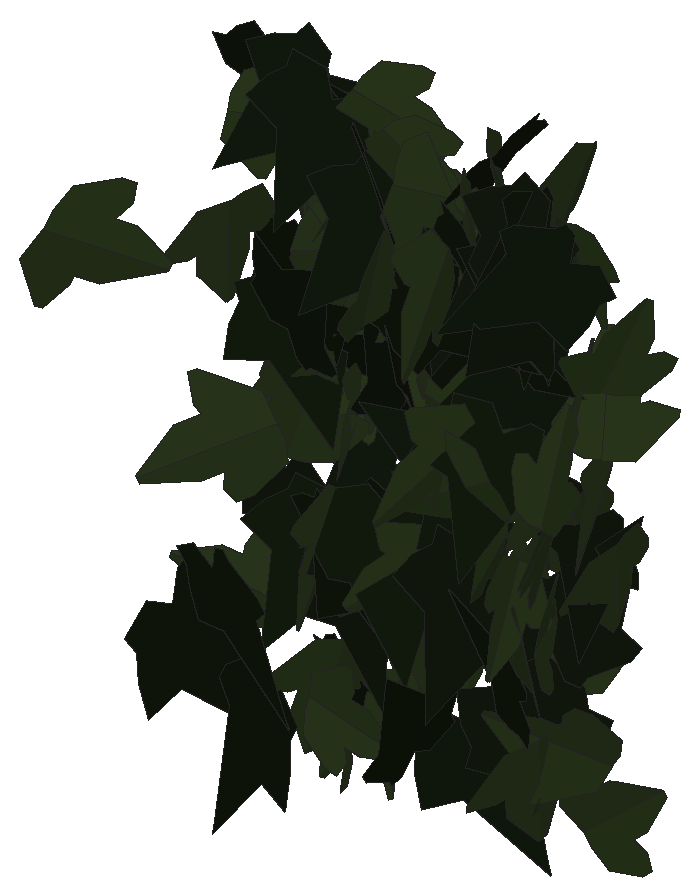
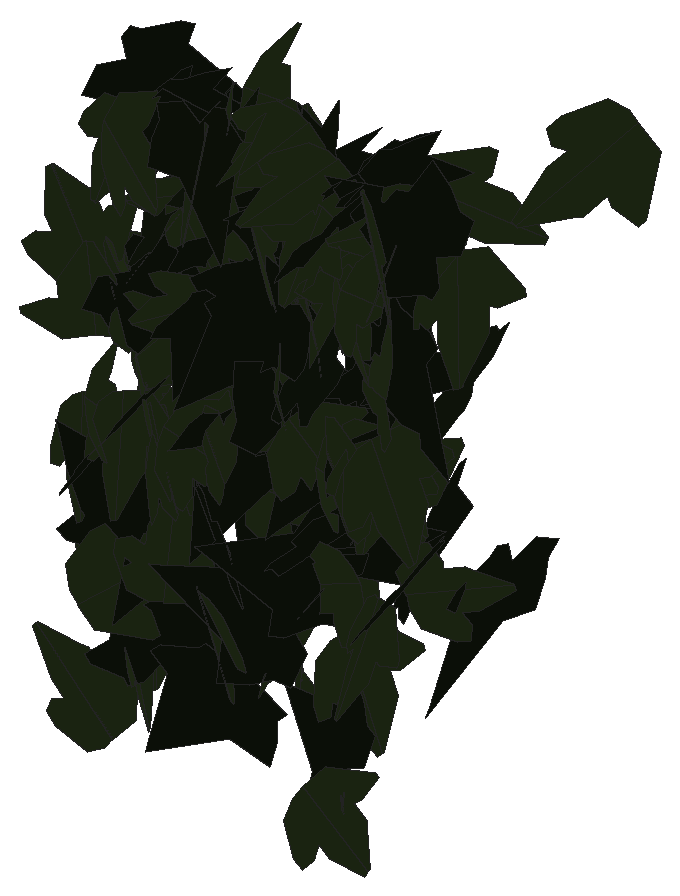
# SketchUp Ruby script. Lengths in inches.
U = 1.inch
M = Sketchup.active_model
def pt(a) = Geom::Point3d.new(a.map { |v| v * U })
def face(e, loops, mat)
  f = e.add_face(loops[0].map { |a| pt(a) })
  loops[1..].each { |l| e.add_face(l.map { |a| pt(a) }).erase! }
  f.material = f.back_material = mat if mat
  f
end
# faces: each face lists its corners as indices into pts; further lists are holes
def faces(e, pts, list, mat = nil) = list.each { |f| face(e, (f[0].is_a?(Array) ? f : [f]).map { |l| l.map { |i| pts[i] } }, mat) }
# xy, xz, yz: faces in a plane at the given z, y or x. An outline is a flat list of corners, or four numbers for a rectangle; further outlines are holes
def ring(l) = l.size == 4 ? [[l[0], l[1]], [l[2], l[1]], [l[2], l[3]], [l[0], l[3]]] : l.each_slice(2).to_a
def flat(e, list, mat, &to3) = list.each { |f| face(e, (f[0].is_a?(Array) ? f : [f]).map { |l| ring(l).map { |u, v| to3.(u, v) } }, mat) }
def xy(e, z, list, mat = nil) = flat(e, list, mat) { |x, y| [x, y, z] }
def xz(e, y, list, mat = nil) = flat(e, list, mat) { |x, z| [x, y, z] }
def yz(e, x, list, mat = nil) = flat(e, list, mat) { |y, z| [x, y, z] }
def lines(e, pts, list) = list.each { |a, b| e.add_line(pt(pts[a]), pt(pts[b])) }
# prism: a flat outline (further loops are holes) pulled along v
def prism(e, loops, v, mat = nil)
  f = face(e, loops, mat); d = Geom::Vector3d.new(v.map { |x| x * U })
  f.pushpull(f.normal.samedirection?(d) ? d.length : -d.length)
end
def box(e, o, s, mat = nil) = prism(e, [[o, [o[0] + s[0], o[1], o[2]], [o[0] + s[0], o[1] + s[1], o[2]], [o[0], o[1] + s[1], o[2]]]], [0, 0, s[2]], mat)
def at(x, y, z, deg = 0) = Geom::Transformation.translation(pt([x, y, z])) * Geom::Transformation.rotation(ORIGIN, Z_AXIS, deg.degrees)
def axes(o, x, y, z) = Geom::Transformation.new([*x, 0, *y, 0, *z, 0, *pt(o).to_a, 1])
def part(name) = M.definitions.add(name)
# library, detail: a bought-in or finely detailed component or shape, given as its bounding box
def library(name, o, s) = part(name).tap { |d| box(d.entities, o, s) }
def detail(e, o, s) = box(e.add_group.entities, o, s)
def put(e, d, t, mat = nil) = e.add_instance(d, t).tap { |i| i.material = mat if mat }
def group(e, t, mat = nil) = e.add_group.tap { |g| g.transformation = t; g.material = mat if mat }.entities
root = M.entities
M.materials.add("efeu1").color = [18, 25, 13]
M.materials.add("efeu2").color = [43, 57, 29]
c1 = part("ivyleaf_10")
p = [[0,0.5,-0.03],[-0.0625,2.02,-0.43],[-0.19,2.01,-0.46],[-0.54,1.05,-0.29],[-0.52,0.625,-0.18],[-0.83,0.76,-0.28],
  [-1.16,0.64,-0.33],[-1.15,0.33,-0.24],[-0.77,-0.39,0.02],[-0.3,-0.51,0.16],[0.04,-0.48,0.23],[-0.02,2.01,-0.4375],
  [-0.06,2.01,-0.43],[0.04,-0.49,0.23],[0.67,-0.49,0.14],[1.38,0.36,-0.2],[1.375,0.51,-0.24],[0.81,0.65,-0.19],
  [0.62,0.59,-0.15],[0.6,1.09,-0.28],[0.5,1.23,-0.31]]
faces(c1.entities,p,[[0,1,2,3,4,5,6,7,8,9,10],[11,12,0,13,14,15,16,17,18,19,20]],"efeu2")
c2 = part("ivyleaf_9")
p = [[1.54,2.16,1.25],[1.36,2.04,1.19],[-0.21,0.99,0.68],[-0.71,1.11,0.82],[-0.85,0.86,0.67],[-0.8,0.17,0.21],
  [-0.9,-0.01,0.1],[-0.67,-0.16,-0.02],[-0.08,-0.08,-0.05],[-0.03,-0.6,-0.4],[0.65,-0.88,-0.66],[0.83,-0.6,-0.49],
  [1.29,-0.42,-0.43],[1.8125,-0.07,-0.26],[1.21,0.44,0.15]]
faces(c2.entities,p,[[0,1,2,3,4,5,6,7,8,9,10,11,12,13,14]],"efeu1")
put(root,c1,axes([527.41,129.42,180.43],[-0.32518,-0.15247,0.84845],[-0.53013,-0.67969,-0.32533],[0.67976,-0.60302,0.15216]))
put(root,c2,axes([526.49,129.75,177.46],[0.55857,-0.71655,0.03403],[0.02142,-0.02645,-0.90854],[0.71704,0.55898,0.00063]))
put(root,c2,axes([526.71,130.62,174.9],[0.21927,-0.17934,-0.93924],[0.70617,-0.61934,0.28311],[-0.64472,-0.73937,-0.00933]))
put(root,c1,axes([523.77,129.47,182.67],[-0.35518,-0.42275,-0.82011],[0.53108,0.62493,-0.55215],[0.75449,-0.6389,0.00258]))
put(root,c1,axes([529.14,131.85,182.77],[-0.01286,-0.49305,0.76391],[0.44109,-0.67144,-0.42595],[0.79505,0.36454,0.24867]))
put(root,c2,axes([528.87,131.65,174.39],[0.24289,0.34244,0.63851],[-0.35118,-0.5334,0.41966],[0.63374,-0.42682,-0.01217]))
put(root,c1,axes([529.3,132.11,179.68],[-0.03772,-0.35118,0.79561],[0.03726,-0.79628,-0.34971],[0.86887,0.0189,0.04954]))
put(root,c2,axes([524.5,131.26,175.47],[0.28969,-0.5067,-0.76251],[-0.37111,0.66613,-0.58364],[0.83693,0.47076,0.00513]))
put(root,c1,axes([529.81,131.96,179.26],[-0.41254,-0.12179,0.76212],[-0.73922,-0.18605,-0.42987],[0.22185,-0.84641,-0.01517]))
put(root,c1,axes([526.91,131.92,174.23],[0.1049,0.03854,0.74126],[0.72695,0.14594,-0.11046],[-0.14999,0.73428,-0.01695]))
put(root,c1,axes([527.66,132.14,181.54],[0.01458,-0.75101,-0.08197],[0.00317,-0.08192,0.75115],[-0.75546,-0.01484,0.00157]))
put(root,c2,axes([529.8,132.64,179.75],[-0.34229,-0.72229,-0.01541],[0.00393,0.01519,-0.79928],[0.72244,-0.3423,-0.00295]))
put(root,c1,axes([530.18,132.5625,177.34],[0.0409,0.59628,-0.475],[-0.03328,-0.47383,-0.59769],[-0.76162,0.05273,0.00061]))
put(root,c1,axes([526.38,132.72,177.13],[0.20032,-0.68078,0.51492],[0.26377,-0.45365,-0.70239],[0.81181,0.31539,0.10116]))
put(root,c2,axes([530.94,132.8125,183.15],[-0.03571,-0.07267,-0.76744],[-0.13202,-0.75633,0.07776],[-0.75948,0.13489,0.02257]))
put(root,c2,axes([529.05,132.98,176.75],[-0.1738,-0.80386,0.29707],[-0.05274,-0.29251,-0.82238],[0.85538,-0.18137,0.00965]))
put(root,c1,axes([525.05,132.65,175.39],[0.19656,0.13798,0.69312],[-0.57621,-0.38526,0.2401],[0.40919,-0.60879,0.00515]))
put(root,c2,axes([529.85,133.16,181.98],[-0.20965,-0.53927,0.62119],[0.02087,-0.64433,-0.55231],[0.82235,-0.12113,0.17239]))
put(root,c2,axes([530.07,132.68,175.26],[0.21332,-0.68005,0.27052],[-0.05728,0.2654,0.71235],[-0.72964,-0.21966,0.02316]))
put(root,c2,axes([526.27,133.19,176.25],[-0.07891,-0.48877,0.70375],[0.14001,-0.70458,-0.47365],[0.84531,0.07108,0.14414]))
put(root,c2,axes([527.08,133.25,182.48],[-0.34583,-0.60775,0.4634],[-0.12688,-0.45592,-0.69263],[0.75365,-0.35563,0.09603]))
put(root,c2,axes([525.41,132.92,180.11],[-0.25145,0.02371,0.8195],[0.4664,-0.70082,0.16338],[0.67426,0.49362,0.1926]))
put(root,c1,axes([530.21,132.75,175.6],[-0.67654,0.37459,0.1769],[0.15072,-0.09297,0.77328],[0.38587,0.69308,0.00812]))
put(root,c1,axes([527.69,133.32,176.61],[-0.05182,-0.31934,0.67271],[-0.16909,-0.65167,-0.32238],[0.7252,-0.17477,-0.02709]))
put(root,c2,axes([527.92,132.6,181.71],[0.1428,0.07843,-0.84206],[0.61962,0.57151,0.1583],[0.57558,-0.63469,0.03849]))
put(root,c1,axes([530.5625,132.86,178.17],[0.30633,-0.69715,-0.10742],[-0.04415,0.09793,-0.76148],[0.70399,0.30949,-0.00102]))
put(root,c1,axes([530.85,132.39,179.09],[0.03357,0.59128,-0.48542],[0.04784,0.48331,0.59202],[0.76351,-0.05628,-0.01575]))
put(root,c2,axes([527.09,133.43,180.13],[0.06108,-0.26606,0.77227],[0.17975,-0.75106,-0.27297],[0.79679,0.18983,0.00239]))
put(root,c1,axes([529.98,133.47,178.53],[-0.04596,0.19222,0.7632],[0.13301,-0.75161,0.19731],[0.77572,0.14026,0.01138]))
put(root,c2,axes([528.67,133.44,182.21],[0.15351,-0.58562,0.55405],[0.21399,-0.51418,-0.60276],[0.77726,0.25722,0.05652]))
put(root,c1,axes([524.18,132.92,181.58],[-0.25348,-0.82349,-0.10141],[0.03287,0.09598,-0.86161],[0.82906,-0.25558,0.00316]))
put(root,c2,axes([527.25,133.14,177.23],[-0.3073,-0.7536,-0.39936],[0.16105,0.36559,-0.81379],[0.83754,-0.34681,0.00995]))
put(root,c2,axes([529.86,133.56,183.02],[-0.42279,-0.51969,0.3609],[-0.1893,-0.31028,-0.66856],[0.60374,-0.46123,0.04311]))
put(root,c1,axes([530.76,132.52,176.46],[-0.02787,0.11799,0.75725],[-0.52626,0.54791,-0.10474],[-0.55714,-0.52345,0.06105]))
put(root,c1,axes([530.24,132.96,174.125],[-0.23443,-0.86981,-0.17617],[0.02648,0.17527,-0.90063],[0.88708,-0.2351,-0.01967]))
put(root,c2,axes([525.73,133.53,176.4],[-0.45283,-0.61602,0.09287],[-0.04067,-0.08533,-0.76435],[0.62165,-0.45432,0.01764]))
put(root,c1,axes([530.87,133.42,174.13],[-0.4028,-0.0512,-0.76261],[-0.69714,-0.32881,0.39029],[-0.31337,0.79731,0.11198]))
put(root,c2,axes([526.57,133.63,182.68],[0.13874,-0.35581,0.72277],[0.23203,-0.68469,-0.3816],[0.77147,0.26991,-0.01521]))
put(root,c1,axes([526,133.34,174.21],[-0.25301,-0.79026,0.19399],[-0.03494,-0.19241,-0.8294],[0.81297,-0.25421,0.02473]))
put(root,c2,axes([526.18,133.42,175.75],[0.26533,-0.75038,-0.0322],[-0.00195,0.03346,-0.79585],[0.75107,0.26517,0.00931]))
put(root,c1,axes([526.82,133.52,173.66],[0.51984,-0.21967,0.46904],[0.42379,-0.20163,-0.56412],[0.29775,0.6705,-0.01597]))
put(root,c2,axes([529.6875,133.93,182.85],[0.07526,-0.24162,-0.73314],[0.37389,-0.63303,0.24701],[-0.67534,-0.3774,0.05505]))
put(root,c1,axes([528.3,133.7,182.87],[0.17681,-0.2807,0.67421],[0.59399,-0.3483,-0.30079],[0.42489,0.60374,0.13994]))
put(root,c2,axes([525.36,133.95,183.55],[-0.25212,-0.72096,0.24078],[-0.04237,-0.23995,-0.76286],[0.75892,-0.25291,0.0374]))
put(root,c1,axes([530.09,133.48,178.02],[0.39837,-0.81768,-0.10342],[-0.03728,0.09687,-0.90952],[0.82335,0.40002,0.00886]))
put(root,c1,axes([525.07,133.48,177.73],[-0.60973,-0.62896,0.18263],[0.12417,0.13398,0.87599],[-0.64306,0.62224,-0.00402]))
put(root,c1,axes([528.7,134.01,177],[-0.03987,-0.04323,0.82819],[0.48947,-0.67056,-0.01144],[0.66947,0.48769,0.05769]))
put(root,c1,axes([526.31,133.45,180.84],[-0.6053,-0.5947,0.31322],[0.22714,0.21573,0.84855],[-0.6326,0.6465,0.00498]))
put(root,c2,axes([524.96,134.18,183.64],[-0.35741,-0.50814,0.46153],[-0.27861,-0.36817,-0.62111],[0.62737,-0.45299,-0.0129]))
put(root,c2,axes([528.25,133.31,180.88],[0.07932,0.10384,-0.80539],[0.4976,0.63329,0.13066],[0.64174,-0.50388,-0.00176]))
put(root,c2,axes([524.9,133.77,180.03],[-0.1353,-0.70648,-0.3928],[0.14631,0.37029,-0.71638],[0.79498,-0.18839,0.06499]))
put(root,c1,axes([527.58,133.17,183.21],[0.06778,-0.45707,-0.70584],[0.35803,0.65642,-0.39069],[0.76088,-0.26816,0.24671]))
put(root,c2,axes([529.72,134.21,180.31],[-0.06714,-0.08179,-0.85804],[-0.24143,-0.8244,0.09748],[-0.82743,0.24718,0.04119]))
put(root,c1,axes([527.02,133.7,183.54],[-0.54247,-0.07339,-0.4915],[0.49257,0.01699,-0.54618],[0.06584,-0.73181,0.03661]))
put(root,c1,axes([527.64,133.72,179.75],[0.66039,-0.34254,0.078],[-0.05548,0.0623,0.74336],[-0.3469,-0.66206,0.0296]))
put(root,c2,axes([528.98,134.31,181.7],[0.22256,-0.64511,0.45029],[0.17516,-0.41559,-0.68196],[0.76697,0.28211,0.02508]))
put(root,c2,axes([528.39,134.26,177.61],[-0.26693,-0.84508,-0.18534],[-0.05178,-0.17801,0.88623],[-0.86361,0.27188,0.00415]))
put(root,c2,axes([525.07,133.77,180.64],[0.24414,0.10742,-0.85145],[-0.78577,-0.32795,-0.26668],[-0.34506,0.82281,0.00487]))
put(root,c1,axes([528.6,133.8,182],[-0.25106,-0.13216,-0.68773],[0.69984,-0.02029,-0.25158],[0.02593,-0.73184,0.13117]))
put(root,c1,axes([530.26,133.73,179.28],[0.47243,-0.64562,0.27146],[-0.16721,0.21399,0.79996],[-0.68011,-0.50108,-0.00812]))
put(root,c1,axes([527.11,133.85,173.92],[-0.20857,0.73523,0.02383],[-0.02107,-0.03073,0.76371],[0.73531,0.20767,0.02865]))
put(root,c2,axes([524.32,134.21,176.51],[0.27125,-0.75607,0.00052],[0.00011,-0.00051,-0.80326],[0.75607,0.27125,-0.00007]))
put(root,c2,axes([527.81,133.59,177.88],[0.65273,0.46953,-0.12028],[-0.10145,-0.06494,-0.80403],[-0.47396,0.66053,0.00645]))
put(root,c1,axes([529.9375,134.02,173.55],[0.28991,-0.71346,-0.09655],[-0.03309,0.09078,-0.77011],[0.7192,0.29178,0.00349]))
put(root,c1,axes([525.49,134.22,178.6],[0.48937,0.15099,-0.52077],[-0.49645,-0.15732,-0.51212],[-0.21803,0.69709,-0.00278]))
put(root,c1,axes([527.15,134.22,181.68],[0.3887,-0.61438,0.09714],[0.05929,-0.07743,-0.72697],[0.61918,0.3931,0.00863]))
put(root,c2,axes([527.82,134.53,181.81],[-0.29098,-0.73419,0.07749],[-0.01443,-0.07762,-0.78961],[0.73813,-0.29094,0.01511]))
put(root,c2,axes([525.34,134.39,172.97],[0.21452,-0.24364,0.69908],[0.42531,-0.55518,-0.324],[0.60595,0.47592,-0.02008]))
put(root,c2,axes([528.01,134.08,173.36],[-0.217,-0.29265,-0.81068],[0.62684,0.52017,-0.35557],[0.59153,-0.65857,0.0794]))
put(root,c1,axes([524.57,134.22,182.56],[-0.34892,0.64965,-0.37007],[0.18173,-0.32245,-0.73739],[-0.72524,-0.39335,-0.00673]))
put(root,c1,axes([525.51,134.25,176.14],[-0.32498,0.07335,-0.64823],[0.58081,-0.29725,-0.32481],[-0.29707,-0.66141,0.07409]))
put(root,c1,axes([530.1875,134.0625,182.76],[-0.66315,0.26247,-0.12788],[0.11183,-0.06482,-0.71295],[-0.2697,-0.67225,0.01881]))
put(root,c1,axes([524.04,133.78,183.04],[-0.10966,-0.17209,-0.79953],[0.71537,0.37077,-0.17793],[0.39636,-0.7168,0.09992]))
put(root,c1,axes([525.51,133.72,181.47],[0.10307,0.77011,0.44627],[0.01116,0.4481,-0.77584],[-0.89,0.0948,0.04195]))
put(root,c1,axes([525.51,134.61,178.32],[0.20734,-0.39803,0.60911],[0.35509,-0.49747,-0.44594],[0.6351,0.40808,0.05048]))
put(root,c1,axes([526.29,133.97,180.09],[0.57482,-0.32089,0.32932],[-0.25992,0.20812,0.65648],[-0.37929,-0.62893,0.04921]))
put(root,c2,axes([525.91,134.8,176.96],[-0.33577,-0.51469,0.48266],[-0.16187,-0.46408,-0.60748],[0.68678,-0.36102,0.09279]))
put(root,c1,axes([528.37,134.7,177.95],[-0.07199,-0.55796,0.633],[0.03795,-0.63679,-0.55699],[0.84295,-0.01898,0.07913]))
put(root,c2,axes([528.6875,134.73,181.71],[0.12406,-0.7653,0.36632],[0.0474,-0.36339,-0.77522],[0.84713,0.13241,-0.01027]))
put(root,c1,axes([527.77,134.09,179.51],[-0.6255,-0.00544,0.43269],[-0.43265,0.02148,-0.62518],[-0.00775,-0.76027,-0.02076]))
put(root,c2,axes([529.94,134.73,177.42],[0.05323,-0.80719,0.28495],[0.01462,-0.2846,-0.80894],[0.85589,0.05506,-0.00391]))
put(root,c1,axes([525.87,133.75,172.42],[-0.02422,0.02425,-0.72519],[-0.31172,0.65487,0.03231],[0.65522,0.31245,-0.01143]))
put(root,c2,axes([529.84,133.96,175.52],[-0.4214,-0.07863,0.75132],[0.75057,0.05368,0.4266],[-0.08541,0.85975,0.04208]))
put(root,c1,axes([528.42,134.29,181.62],[0.75216,-0.13805,-0.25891],[-0.25365,0.0522,-0.7647],[0.1475,0.79376,0.00526]))
put(root,c1,axes([530.8,134.19,177.27],[-0.07725,-0.77871,-0.18603],[0.03324,0.18361,-0.7824],[0.79993,-0.08283,0.01455]))
put(root,c2,axes([526.4375,134.69,178.89],[0.24623,0.31078,0.78856],[-0.48046,-0.6253,0.39647],[0.69826,-0.53986,-0.00527]))
put(root,c1,axes([525.26,134.44,181.53],[0.22863,-0.70155,0.04792],[0.00071,-0.05016,-0.73772],[0.70318,0.22815,-0.01483]))
put(root,c1,axes([530.69,134.3125,180.44],[-0.36465,-0.64345,0.18972],[0.10637,0.15775,0.73945],[-0.66235,0.37958,0.0143]))
put(root,c1,axes([524.75,134.26,178.6],[-0.44527,-0.55203,-0.14254],[0.09034,0.11026,-0.70922],[0.56293,-0.45434,0.00107]))
put(root,c1,axes([524.77,134.88,181.93],[-0.02649,-0.45044,0.65683],[0.34696,-0.59808,-0.39616],[0.7169,0.27281,0.216]))
put(root,c2,axes([529.27,134.11,173.44],[-0.54558,-0.27228,0.60432],[0.56111,0.22693,0.60881],[-0.35284,0.7819,0.03375]))
put(root,c1,axes([530.04,134.84,178.11],[0.20891,-0.4049,0.58719],[0.33907,-0.48192,-0.45295],[0.62751,0.3952,0.04926]))
put(root,c2,axes([525.49,134.03,179.16],[0.74907,0.35719,-0.05557],[-0.05144,-0.02122,-0.82987],[-0.35781,0.75083,0.00298]))
put(root,c2,axes([526.03,133.96,175.85],[0.11724,0.05004,0.79873],[0.72405,0.33725,-0.12741],[-0.34092,0.73347,0.00409]))
put(root,c1,axes([529.88,134.33,177.68],[-0.15936,-0.75624,-0.21444],[0.04192,0.21031,-0.77285],[0.78494,-0.16477,-0.00227]))
put(root,c2,axes([523.45,134.55,183.02],[0.25635,-0.15699,0.75804],[0.65262,-0.38565,-0.30057],[0.41636,0.70115,0.0044]))
put(root,c2,axes([525.85,134.89,179.74],[0.56315,-0.67128,0.12791],[-0.05325,0.12214,0.87542],[-0.68128,-0.56443,0.03731]))
put(root,c1,axes([524.48,134.89,178.7],[-0.13367,-0.58614,0.47424],[-0.12219,-0.45842,-0.60103],[0.74399,-0.1806,-0.01351]))
put(root,c1,axes([530.23,134.51,172.21],[-0.58229,-0.11113,0.63829],[0.62406,0.13437,0.59271],[-0.17407,0.85347,-0.01021]))
put(root,c2,axes([525.33,134.95,182.9],[-0.01297,-0.76983,0.10528],[-0.00435,-0.10522,-0.76993],[0.77698,-0.01344,-0.00255]))
put(root,c1,axes([524.11,134.9,180.35],[0.1211,-0.23441,0.79724],[0.73806,-0.33987,-0.21204],[0.38185,0.73127,0.15701]))
put(root,c1,axes([528.72,134.74,175.35],[-0.50846,-0.52162,-0.13871],[-0.08411,-0.11166,0.72823],[-0.53315,0.51507,0.01739]))
put(root,c1,axes([525.77,134.92,179],[-0.25663,-0.595,0.42459],[-0.01871,-0.4445,-0.63422],[0.73072,-0.22035,0.13288]))
put(root,c1,axes([525.66,134.46,178.82],[0.51872,-0.29665,-0.41728],[-0.33142,0.25821,-0.59555],[0.39024,0.61362,0.04888]))
put(root,c1,axes([526.75,134.58,179.64],[0.72391,0.28758,0.14692],[0.13832,0.04974,-0.77892],[-0.29181,0.73699,-0.00476]))
put(root,c2,axes([527.71,134.8,176.7],[-0.45768,0.04819,-0.63271],[0.63268,-0.0251,-0.45957],[-0.0486,-0.78049,-0.02429]))
put(root,c1,axes([526.24,134.92,179.64],[0.193,-0.19282,0.66763],[0.57952,-0.33772,-0.26507],[0.3835,0.60739,0.06456]))
put(root,c1,axes([524.27,134.79,178.96],[-0.22593,-0.81988,0.2014],[-0.05977,-0.19243,-0.85042],[0.84214,-0.23362,-0.00633]))
put(root,c1,axes([524.86,134.25,175.64],[0.08175,-0.60823,-0.51662],[0.11729,0.52284,-0.597],[0.78936,-0.0147,0.14221]))
put(root,c2,axes([528.32,134.34,183.49],[-0.13304,0.74721,-0.05839],[0.01253,-0.05708,-0.75896],[-0.74938,-0.1336,-0.00233]))
put(root,c1,axes([530.41,134.42,179.33],[0.67659,0.4743,-0.08218],[0.0506,0.0709,0.82577],[0.4787,-0.67786,0.02887]))
put(root,c1,axes([524.64,134.57,183.26],[0.47245,-0.6454,-0.29145],[-0.15137,0.25022,-0.79948],[0.69179,0.49552,0.02411]))
put(root,c1,axes([528.08,134.64,180.47],[-0.34312,-0.10859,-0.60991],[0.61912,-0.08462,-0.33324],[-0.02178,-0.69466,0.13594]))
put(root,c2,axes([527.69,134.65,180.68],[0.00637,-0.64745,-0.45045],[-0.02825,0.44999,-0.64719],[0.78823,0.02136,-0.01956]))
put(root,c1,axes([527.4,134.93,177.9],[-0.26989,0.01283,0.68452],[0.64093,-0.25394,0.25747],[0.24069,0.69059,0.08196]))
put(root,c1,axes([525.88,134.59,182.68],[-0.70512,0.14114,-0.10133],[0.1023,-0.00507,-0.71895],[-0.14044,-0.71235,-0.01496]))
put(root,c1,axes([525.84,134.46,183.59],[-0.33069,-0.33628,-0.58463],[0.54687,0.24739,-0.45163],[0.39474,-0.62446,0.13591]))
put(root,c1,axes([528.27,134.47,183.2],[-0.52264,0.53881,0.21262],[-0.17208,0.12902,-0.74994],[-0.55309,-0.54928,0.03241]))
put(root,c1,axes([527.71,134.86,175.13],[0.72407,-0.4739,0.08186],[0.06643,-0.04799,-0.86535],[0.47631,0.7271,-0.00376]))
put(root,c1,axes([529.35,135.125,183.28],[0.24043,-0.75117,0.41228],[0.15348,-0.38353,-0.78829],[0.84302,0.28406,0.02593]))
put(root,c1,axes([529.8125,135,174.84],[-0.39945,-0.12453,-0.69293],[-0.66012,-0.21074,0.41841],[-0.24477,0.77156,0.00244]))
put(root,c2,axes([526.51,134.45,175.14],[0.52092,0.35781,-0.5095],[0.26796,0.47078,0.60459],[0.56197,-0.55616,0.18399]))
put(root,c2,axes([526.8,134.32,180.79],[0.66156,0.41069,0.14511],[0.11381,0.09173,-0.77847],[-0.42044,0.67105,0.01761]))
put(root,c1,axes([529.24,134.41,177.33],[-0.03802,0.07536,0.85124],[-0.76508,0.3766,-0.06751],[-0.38071,-0.76435,0.05066]))
put(root,c1,axes([525.3,135.13,172.55],[-0.16127,-0.62162,0.40611],[-0.08962,-0.39624,-0.6421],[0.73709,-0.18418,0.01078]))
